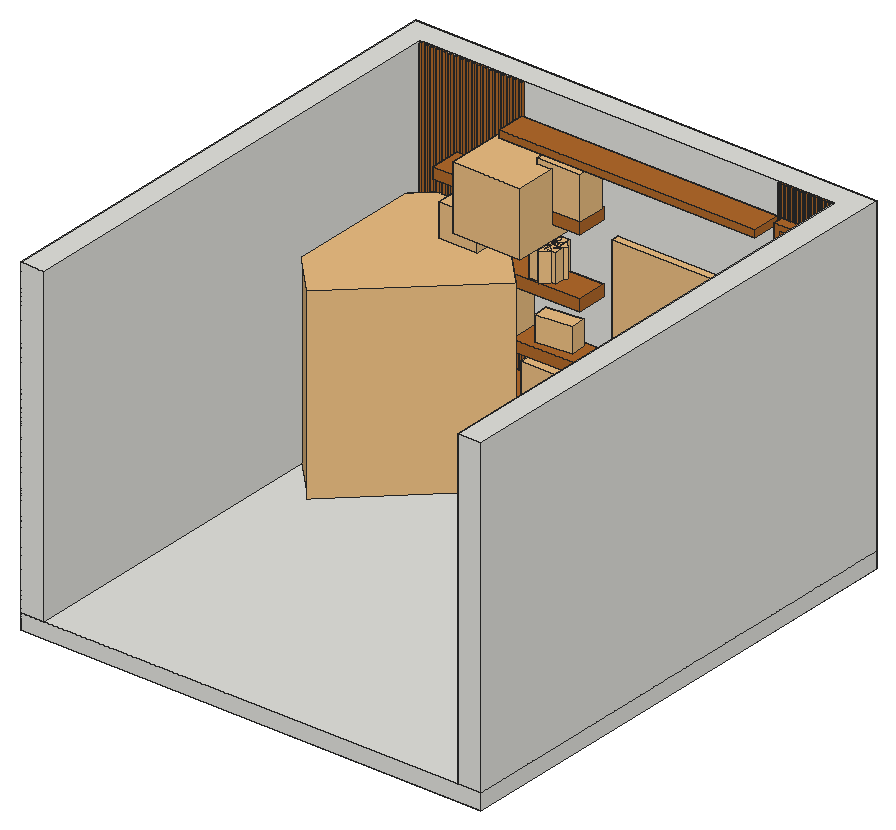
# SketchUp Ruby script. Lengths in inches.
U = 1.inch
M = Sketchup.active_model
def pt(a) = Geom::Point3d.new(a.map { |v| v * U })
def face(e, loops, mat)
  f = e.add_face(loops[0].map { |a| pt(a) })
  loops[1..].each { |l| e.add_face(l.map { |a| pt(a) }).erase! }
  f.material = f.back_material = mat if mat
  f
end
# faces: each face lists its corners as indices into pts; further lists are holes
def faces(e, pts, list, mat = nil) = list.each { |f| face(e, (f[0].is_a?(Array) ? f : [f]).map { |l| l.map { |i| pts[i] } }, mat) }
# xy, xz, yz: faces in a plane at the given z, y or x. An outline is a flat list of corners, or four numbers for a rectangle; further outlines are holes
def ring(l) = l.size == 4 ? [[l[0], l[1]], [l[2], l[1]], [l[2], l[3]], [l[0], l[3]]] : l.each_slice(2).to_a
def flat(e, list, mat, &to3) = list.each { |f| face(e, (f[0].is_a?(Array) ? f : [f]).map { |l| ring(l).map { |u, v| to3.(u, v) } }, mat) }
def xy(e, z, list, mat = nil) = flat(e, list, mat) { |x, y| [x, y, z] }
def xz(e, y, list, mat = nil) = flat(e, list, mat) { |x, z| [x, y, z] }
def yz(e, x, list, mat = nil) = flat(e, list, mat) { |y, z| [x, y, z] }
def lines(e, pts, list) = list.each { |a, b| e.add_line(pt(pts[a]), pt(pts[b])) }
# prism: a flat outline (further loops are holes) pulled along v
def prism(e, loops, v, mat = nil)
  f = face(e, loops, mat); d = Geom::Vector3d.new(v.map { |x| x * U })
  f.pushpull(f.normal.samedirection?(d) ? d.length : -d.length)
end
def box(e, o, s, mat = nil) = prism(e, [[o, [o[0] + s[0], o[1], o[2]], [o[0] + s[0], o[1] + s[1], o[2]], [o[0], o[1] + s[1], o[2]]]], [0, 0, s[2]], mat)
def at(x, y, z, deg = 0) = Geom::Transformation.translation(pt([x, y, z])) * Geom::Transformation.rotation(ORIGIN, Z_AXIS, deg.degrees)
def axes(o, x, y, z) = Geom::Transformation.new([*x, 0, *y, 0, *z, 0, *pt(o).to_a, 1])
def part(name) = M.definitions.add(name)
# library, detail: a bought-in or finely detailed component or shape, given as its bounding box
def library(name, o, s) = part(name).tap { |d| box(d.entities, o, s) }
def detail(e, o, s) = box(e.add_group.entities, o, s)
def put(e, d, t, mat = nil) = e.add_instance(d, t).tap { |i| i.material = mat if mat }
def group(e, t, mat = nil) = e.add_group.tap { |g| g.transformation = t; g.material = mat if mat }.entities
root = M.entities
M.materials.add("Material__1").color = [95, 70, 46]
M.materials.add("[Color M09]").color = [0, 0, 0]
M.materials.add("[Color_009]").color = [0, 0, 0]
M.materials.add("[Metal_Corrogated_Shiny]1").color = [193, 193, 193]
M.materials.add("[Wood Bamboo]").color = [177, 105, 43]
M.materials.add("wire_5").color = [232, 232, 232]
c1 = library("TV WALL",[28.53,10.9,29.38],[49.35,7.98,28.84])
c2 = library("Palm",[82.2,-9.29,-2.36],[51.18,55.77,65.42])
c3 = library("Pinch Pot",[-27.95,-27.95,0],[55.9,55.9,47.42])
c4 = library("Group\#386",[-915.9375,-34.5,735.6],[41.04,40.85,6.81])
c5 = library("Group\#403",[-912.1,-32.49,735.82],[33.14,36.63,9.55])
c6 = part("Potted palm")
put(c6.entities,c2,axes([3796.42,-10488.37,43.97],[0,116.51338,0],[-116.51338,0,0],[0,0,116.51338]))
put(c6.entities,c3,axes([1647.67,1801.1875,0],[0,30.58476,0],[-30.58476,0,0],[0,0,45.1095]))
put(c6.entities,c4,axes([32580.48,2279.8125,-23417.78],[34.48768,0,0],[0,34.48768,0],[0,0,34.48768]),"Material__1")
put(c6.entities,c5,axes([32580.48,2279.8125,-23417.78],[34.48768,0,0],[0,34.48768,0],[0,0,34.48768]),"wire_5")
c7 = part("Sem+nome (1)")
p = [[29.74,41.24,0.13],[30.16,40.82,0.13],[30.16,41.24,0.13]]
lines(c7.entities,p,[[0,1],[1,2],[2,0]])
put(c7.entities,c6,axes([-218.92,51.09,-6.7],[0.00697,0.0066,0],[0.0066,-0.00697,0],[0,0,0.0096]))
c8 = library("House Plant - small",[0,0,0],[36.52,33.08,30.88])
c9 = library("decor3\#1",[2.52,2.29,3.29],[10.02,10.5,11.12])
c10 = library("14",[-2.11,-5.07,0],[5.66,13.58,9.28])
c11 = library("Flowers",[-19.1,-13.04,-3.93],[34.91,25.83,49.88])
c12 = library("6",[0,0,0],[30.12,28.16,55.56])
c13 = library("Flowers\#1",[-13.99,-28.13,0.53],[25.34,35.06,49.37])
c14 = library("Fluted vase segment",[0,0,0.06],[101.29,86.53,393.7])
c15 = part("vase corigated")
xy(c15.entities,0,[[0,-99.44,-25.74,-96.05,-49.72,-86.12,-70.32,-70.32,-86.12,-49.72,-96.05,-25.74,-99.44,0,-96.05,25.74,-86.12,49.72,-70.32,70.32,-49.72,86.12,-25.74,96.05,0,99.44,25.74,96.05,49.72,86.12,70.32,70.32,86.12,49.72,96.05,25.74,99.44,0,96.05,-25.74,86.12,-49.72,70.32,-70.32,49.72,-86.12,25.74,-96.05]],"[Color_009]")
put(c15.entities,c14,at(27.84,-86.53,-0.06),"[Metal_Corrogated_Shiny]1")
put(c15.entities,c14,at(80.87,-41.5,-0.06,45),"[Metal_Corrogated_Shiny]1")
put(c15.entities,c14,at(86.53,27.84,-0.06,90),"[Metal_Corrogated_Shiny]1")
put(c15.entities,c14,at(41.5,80.87,-0.06,135),"[Metal_Corrogated_Shiny]1")
put(c15.entities,c14,at(-27.84,86.53,-0.06,-180),"[Metal_Corrogated_Shiny]1")
put(c15.entities,c14,at(-80.87,41.5,-0.06,-135),"[Metal_Corrogated_Shiny]1")
put(c15.entities,c14,at(-86.53,-27.84,-0.06,-90),"[Metal_Corrogated_Shiny]1")
put(c15.entities,c14,at(-41.5,-80.87,-0.06,-45),"[Metal_Corrogated_Shiny]1")
c16 = library("Vase-8",[-47.51,-47.51,0],[95.02,95.02,78.375])
c17 = library("Plant+Philodendron+Scandens",[-5.75,-7.35,0],[25.95,25.95,24.43])
put(root,c1,axes([50.76,166.0625,7.66],[1.188,0,0],[0,1,0],[0,0,1.23876]))
put(root,c7,at(220.44,102.58,6.875))
put(root,c8,axes([59.4375,165.25,21.07],[0.36652,0,0],[0,0.275,0],[0,0,0.438]))
put(root,c9,axes([33.03,165.58,34.12],[1.64,0,0],[0,1,0],[0,0,1.4652]))
put(root,c10,at(64.99,174.86,38.9375,-84.3))
put(root,c8,axes([150,169.61,87.14],[0.36652,0,0],[0,0.275,0],[0,0,0.438]))
put(root,c11,axes([145.25,170.875,22.65],[0.4352,0,0],[0,0.3625,0],[0,0,0.462]))
put(root,c9,axes([58.83,166,82.87],[1.64,0,0],[0,1,0],[0,0,1.4652]))
put(root,c12,at(141.62,141.18,0))
put(root,c13,axes([41.95,175.23,61.98],[0.58157,0,0],[0,0.6248,0],[0,0,0.42954]))
put(root,c15,axes([62.78,174.55,61.375],[0.04048,0,0],[0,0.04194,0],[0,0,0.02724]))
put(root,c16,axes([155.89,174.49,60.63],[0.09131,0,0],[0,0.06751,0],[0,0,0.22286]))
put(root,c17,at(48.5,160.59,77.73))
g1 = group(root,at(0,0,0))
xy(g1,0,[[0,0,0,189,176.3125,189,176.3125,0,167.3125,0,167.3125,180,9,180,9,0]])
xy(g1,120,[[0,0,9,0,9,180,167.3125,180,167.3125,0,176.3125,0,176.3125,189,0,189]])
xz(g1,0,[[0,0,9,120],[167.3125,0,176.3125,120]])
xz(g1,180,[[10.3,0,167.3125,120]])
xz(g1,189,[[0,0,176.3125,120]])
yz(g1,0,[[0,0,189,120]])
yz(g1,9,[[0,0,180,120]])
yz(g1,167.3125,[[0,0,180,120]])
yz(g1,176.3125,[[0,0,189,120]])
g2 = group(g1,at(9,180,0),"[Wood Bamboo]")
box(g2,[0,-0.8125,0],[1.3,0.8125,120])
box(g2,[2.25,-0.8125,0],[1.3,0.8125,120])
box(g2,[4.5,-0.8125,0],[1.3,0.8125,120])
box(g2,[6.75,-0.8125,0],[1.3,0.8125,120])
box(g2,[9,-0.8125,0],[1.3,0.8125,120])
box(g2,[11.25,-0.8125,0],[1.3,0.8125,120])
box(g2,[13.5,-0.8125,0],[1.3,0.8125,120])
box(g2,[15.75,-0.8125,0],[1.3,0.8125,120])
box(g2,[18,-0.8125,0],[1.3,0.8125,120])
box(g2,[20.25,-0.8125,0],[1.3,0.8125,120])
box(g2,[22.5,-0.8125,0],[1.3,0.8125,120])
box(g2,[24.75,-0.8125,0],[1.3,0.8125,120])
box(g2,[27,-0.8125,0],[1.3,0.8125,120])
box(g2,[29.25,-0.8125,0],[1.3,0.8125,120])
box(g2,[31.5,-0.8125,0],[1.3,0.8125,120])
box(g2,[33.75,-0.8125,0],[1.3,0.8125,120])
box(g2,[36,-0.8125,0],[1.3,0.8125,120])
box(g2,[38.25,-0.8125,0],[1.3,0.8125,120])
g3 = group(g1,at(140.625,180,0),"[Wood Bamboo]")
box(g3,[8.57,-0.8125,0],[0.98,0.8125,120])
box(g3,[10,-0.8125,0],[0.98,0.8125,120])
box(g3,[11.43,-0.8125,0],[0.98,0.8125,120])
box(g3,[12.86,-0.8125,0],[0.97,0.8125,120])
box(g3,[14.28,-0.8125,0],[0.98,0.8125,120])
box(g3,[15.71,-0.8125,0],[0.98,0.8125,120])
box(g3,[17.14,-0.8125,0],[0.98,0.8125,120])
box(g3,[18.57,-0.8125,0],[0.98,0.8125,120])
box(g3,[20,-0.8125,0],[0.98,0.8125,120])
box(g3,[21.43,-0.8125,0],[0.97,0.8125,120])
box(g3,[22.85,-0.8125,0],[0.98,0.8125,120])
box(g3,[24.28,-0.8125,0],[0.98,0.8125,120])
box(g3,[25.71,-0.8125,0],[0.98,0.8125,120])
box(g3,[7.14,-0.8125,0],[0.98,0.8125,120])
box(g3,[5.71,-0.8125,0],[0.98,0.8125,120])
g4 = group(g1,at(48.55,179.1875,105.99),"[Wood Bamboo]")
box(g4,[0,-10.9375,0],[97.78,10.9375,2.63])
g5 = group(g1,at(23.8,179.1875,84.72),"[Wood Bamboo]")
prism(g5,[[[0,0,-1.3125],[55.44,0.73,-1.3125],[55.59,-10.89,-1.3125],[0.15,-11.62,-1.3125]]],[0,0,4.27])
g6 = group(g1,at(23.8,179.1875,58.41),"[Wood Bamboo]")
prism(g6,[[[0,0,-1.3125],[55.44,0.73,-1.3125],[55.59,-10.89,-1.3125],[0.15,-11.62,-1.3125]]],[0,0,4.27])
g7 = group(g1,at(23.8,179.1875,35.97),"[Wood Bamboo]")
prism(g7,[[[0,0,-1.3125],[55.44,0.73,-1.3125],[55.59,-10.89,-1.3125],[0.15,-11.62,-1.3125]]],[0,0,4.27])
g8 = group(root,at(0,0,120))
box(g8,[0,0,-126],[176.3125,189,6])
g9 = group(root,at(31.5,179.1875,5.36))
xy(g9,0,[[-7.55,-17.1875,134.38,0]])
xy(g9,15.72,[[-7.55,-17.1875,134.38,0]],"[Wood Bamboo]")
xz(g9,-17.1875,[[-7.55,0,27.9375,15.72],[27.9375,0,63.42,15.72],[63.42,0,98.9,15.72],[98.9,0,134.38,15.72]])
xz(g9,0,[[-7.55,0,134.38,15.72]])
yz(g9,-7.55,[[-17.1875,0,0,15.72]],"[Wood Bamboo]")
yz(g9,134.38,[[-17.1875,0,0,15.72]])
g10 = group(root,at(143.21,155.16,47.83))
xy(g10,-9.8125,[[4.9375,20.1875,20.9375,24.625]])
xy(g10,-7.8,[[6.95,20.1875,18.92,22.41]],"[Wood Bamboo]")
xy(g10,10.37,[[6.95,20.1875,18.92,22.41]])
xy(g10,12.8,[[6.95,20.1875,18.92,22.41]],"[Wood Bamboo]")
xy(g10,37.125,[[6.95,20.1875,18.92,22.41]])
xy(g10,39.4,[[6.95,20.1875,18.92,22.41]],"[Wood Bamboo]")
xy(g10,58.77,[[6.95,20.1875,18.92,22.41]])
xy(g10,60.79,[[4.9375,20.1875,20.9375,24.625]],"[Wood Bamboo]")
xz(g10,20.1875,[[[4.9375,-9.8125,20.9375,60.79],[6.95,-7.8,18.92,58.77]],[6.95,10.37,18.92,12.8],[6.95,37.125,18.92,39.4]],"[Wood Bamboo]")
xz(g10,22.41,[[6.95,-7.8,18.92,10.37],[6.95,12.8,18.92,37.125],[6.95,39.4,18.92,58.77]])
xz(g10,24.625,[[4.9375,-9.8125,20.9375,60.79]])
yz(g10,4.9375,[[20.1875,-9.8125,24.625,60.79]],"[Wood Bamboo]")
yz(g10,6.95,[[20.1875,-7.8,22.41,10.37],[20.1875,12.8,22.41,37.125],[20.1875,39.4,22.41,58.77]],"[Wood Bamboo]")
yz(g10,18.92,[[20.1875,-7.8,22.41,10.37],[20.1875,12.8,22.41,37.125],[20.1875,39.4,22.41,58.77]],"[Wood Bamboo]")
yz(g10,20.9375,[[20.1875,-9.8125,24.625,60.79]])
g11 = group(root,at(94.92,174.75,21.07))
xy(g11,0,[[0,0,39.5625,4.4375]])
xy(g11,3.9375,[[0,0,39.5625,4.4375]],"[Color M09]")
xz(g11,0,[[0,0,39.5625,3.9375]],"[Color M09]")
xz(g11,4.4375,[[0,0,39.5625,3.9375]])
yz(g11,0,[[0,0,4.4375,3.9375]],"[Color M09]")
yz(g11,39.5625,[[0,0,4.4375,3.9375]])
